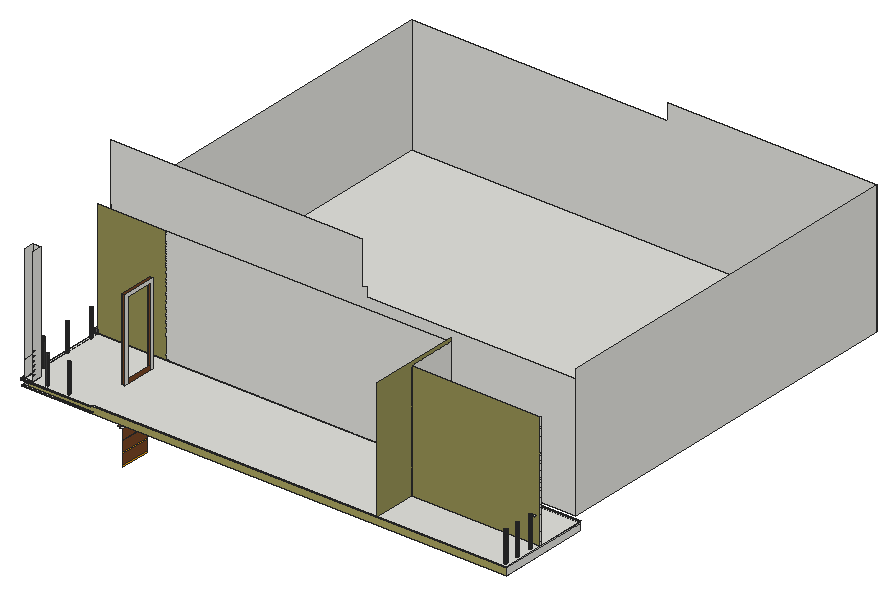
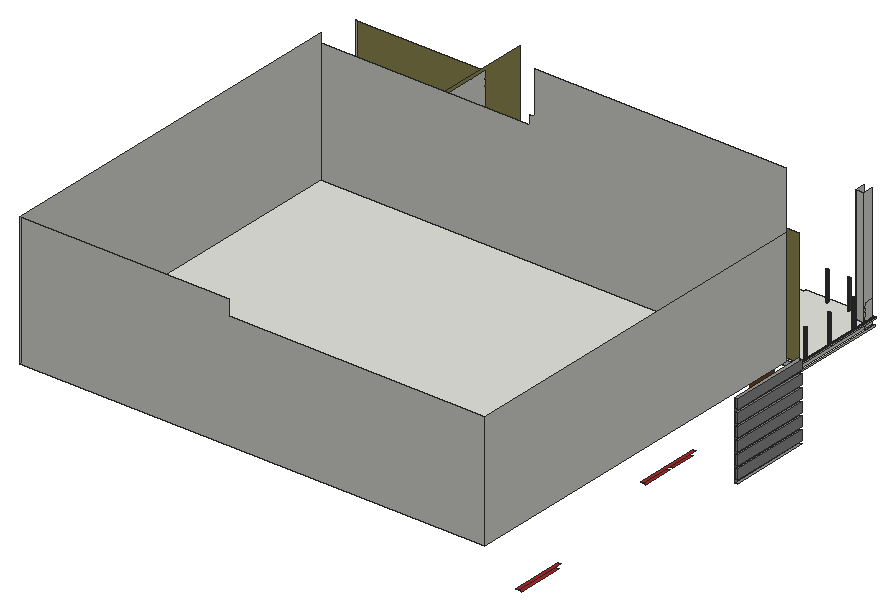
# SketchUp Ruby script. Lengths in inches.
U = 1.inch
M = Sketchup.active_model
def pt(a) = Geom::Point3d.new(a.map { |v| v * U })
def face(e, loops, mat)
  f = e.add_face(loops[0].map { |a| pt(a) })
  loops[1..].each { |l| e.add_face(l.map { |a| pt(a) }).erase! }
  f.material = f.back_material = mat if mat
  f
end
# faces: each face lists its corners as indices into pts; further lists are holes
def faces(e, pts, list, mat = nil) = list.each { |f| face(e, (f[0].is_a?(Array) ? f : [f]).map { |l| l.map { |i| pts[i] } }, mat) }
# xy, xz, yz: faces in a plane at the given z, y or x. An outline is a flat list of corners, or four numbers for a rectangle; further outlines are holes
def ring(l) = l.size == 4 ? [[l[0], l[1]], [l[2], l[1]], [l[2], l[3]], [l[0], l[3]]] : l.each_slice(2).to_a
def flat(e, list, mat, &to3) = list.each { |f| face(e, (f[0].is_a?(Array) ? f : [f]).map { |l| ring(l).map { |u, v| to3.(u, v) } }, mat) }
def xy(e, z, list, mat = nil) = flat(e, list, mat) { |x, y| [x, y, z] }
def xz(e, y, list, mat = nil) = flat(e, list, mat) { |x, z| [x, y, z] }
def yz(e, x, list, mat = nil) = flat(e, list, mat) { |y, z| [x, y, z] }
def lines(e, pts, list) = list.each { |a, b| e.add_line(pt(pts[a]), pt(pts[b])) }
# prism: a flat outline (further loops are holes) pulled along v
def prism(e, loops, v, mat = nil)
  f = face(e, loops, mat); d = Geom::Vector3d.new(v.map { |x| x * U })
  f.pushpull(f.normal.samedirection?(d) ? d.length : -d.length)
end
def box(e, o, s, mat = nil) = prism(e, [[o, [o[0] + s[0], o[1], o[2]], [o[0] + s[0], o[1] + s[1], o[2]], [o[0], o[1] + s[1], o[2]]]], [0, 0, s[2]], mat)
def at(x, y, z, deg = 0) = Geom::Transformation.translation(pt([x, y, z])) * Geom::Transformation.rotation(ORIGIN, Z_AXIS, deg.degrees)
def axes(o, x, y, z) = Geom::Transformation.new([*x, 0, *y, 0, *z, 0, *pt(o).to_a, 1])
def part(name) = M.definitions.add(name)
# library, detail: a bought-in or finely detailed component or shape, given as its bounding box
def library(name, o, s) = part(name).tap { |d| box(d.entities, o, s) }
def detail(e, o, s) = box(e.add_group.entities, o, s)
def put(e, d, t, mat = nil) = e.add_instance(d, t).tap { |i| i.material = mat if mat }
def group(e, t, mat = nil) = e.add_group.tap { |g| g.transformation = t; g.material = mat if mat }.entities
root = M.entities
M.materials.add("[0018_Brown]").color = [165, 42, 42]
M.materials.add("[0038_Orange]").color = [255, 165, 0]
M.materials.add("[0057_DarkKhaki]").color = [150, 145, 85]
M.materials.add("[0134_DimGray]").color = [105, 105, 105]
M.materials.add("[0137_Black]").color = [71, 71, 71]
M.materials.add("[Color M05]").color = [145, 145, 145]
M.materials.add("[Wood Veneer 01]").color = [120, 70, 37]
xy(root,168.28,[[8.875,116.75,11.875,199.5]],"[Color M05]")
xy(root,171.32,[[8.875,116.75,11.875,199.5]],"[Color M05]")
xy(root,181.4,[[8.875,116.75,11.875,199.5]],"[Color M05]")
xy(root,184.44,[[8.875,116.75,11.875,199.5]],"[Color M05]")
xy(root,191.21,[[8.875,431.78,11.875,479.72]],"[0018_Brown]")
xy(root,194.21,[[8.875,428.78,11.875,482.72]],"[0018_Brown]")
xy(root,194.53,[[8.875,116.75,11.875,199.5]],"[Color M05]")
xy(root,197.57,[[8.875,116.75,11.875,199.5]],"[Color M05]")
xy(root,204,[[79.85,61.11,82.85,91.11]])
xy(root,207,[[79.85,58.11,82.85,94.11]],"[Wood Veneer 01]")
xy(root,207.65,[[8.875,116.75,11.875,199.5]],"[Color M05]")
xy(root,210.69,[[8.875,116.75,11.875,199.5]],"[Color M05]")
xy(root,219.65,[[8.875,257.47,11.875,284.27],[8.875,287.91,11.875,318.35]],"[0018_Brown]")
xy(root,220.78,[[8.875,116.75,11.875,199.5]],"[Color M05]")
xy(root,222.65,[[8.875,254.47,11.875,321.35]],"[0018_Brown]")
xy(root,223.82,[[8.875,116.75,11.875,199.5]],"[Color M05]")
xy(root,233.9,[[8.875,116.75,11.875,199.5]],"[Color M05]")
xy(root,235.42,[[9.5625,21.375,9.5625,116.75,510.6875,116.75,510.6875,22.0625,82.9375,22.0625,82.9375,21.375]],"[0057_DarkKhaki]")
xy(root,236.47,[[9.5625,21.375,82.9375,21.375,82.9375,22.0625,11.875,22.0625,11.875,116.75,9.5625,116.75]])
xy(root,236.94,[[8.875,116.75,11.875,199.5]],"[Color M05]")
xy(root,242.04,[[20.875,22.0625,20.875,31.0625,11.875,31.0625,11.875,116.75,510.6875,116.75,510.6875,22.0625]])
xy(root,242.08,[[9.5625,19.6875,9.5625,116.75,11.875,116.75,11.875,22.0625,82.85,22.0625,82.85,19.6875]])
xy(root,243,[[9.5625,19.6875,9.5625,116.75,11.875,116.75,11.875,22.0625,82.85,22.0625,82.85,19.6875],[20.875,22.0625,82.85,22.0625,82.85,63.65,79.85,63.65,79.85,66.65,82.85,66.65,82.85,96.65,79.85,96.65,79.85,99.65,82.85,99.65,82.85,116.75,11.875,116.75,11.875,31.0625,20.875,31.0625],[376.99,22.0625,510.6875,66.25],[79.85,63.65,82.85,66.65],[376.99,66.25,509.75,116.75],
  [509.75,66.25,510.6875,116.75],[79.85,96.65,82.85,99.65],[11.875,116.75,376.99,119.6875],[376.99,116.75,509.75,119.6875],[20.875,122.75,501.6875,511.875]])
xy(root,243.17,[[[9.5625,19.6875,82.85,19.6875,82.85,22.0625,510.6875,22.0625,510.6875,116.75,9.5625,116.75],[11.875,22.0625,20.6875,32.5],[505.89,26.06,505.51,26.11,505.17,26.25,504.87,26.48,504.64,26.78,504.5,27.125,504.45,27.5,504.5,27.87,504.64,28.22,504.87,28.51,505.17,28.74,505.51,28.89,505.89,28.93,506.26,28.89,506.6,28.74,506.9,28.51,507.13,28.22,507.27,27.87,507.32,27.5,507.27,27.125,507.13,26.78,506.9,26.48,506.6,26.25,506.26,26.11],[505.89,40.75,505.51,40.8,505.17,40.9375,504.87,41.17,504.64,41.47,504.5,41.8125,504.45,42.18,504.5,42.56,504.64,42.9,504.87,43.2,505.17,43.43,505.51,43.57,505.89,43.62,506.26,43.57,506.6,43.43,506.9,43.2,507.13,42.9,507.27,42.56,507.32,42.18,507.27,41.8125,507.13,41.47,506.9,41.17,506.6,40.9375,506.26,40.8],[505.89,57.31,505.51,57.36,505.17,57.5,504.87,57.73,504.64,58.03,504.5,58.375,504.45,58.75,504.5,59.12,504.64,59.47,504.87,59.76,505.17,59.99,505.51,60.14,505.89,60.18,506.26,60.14,506.6,59.99,506.9,59.76,507.13,59.47,507.27,59.12,507.32,58.75,507.27,58.375,507.13,58.03,506.9,57.73,506.6,57.5,506.26,57.36],[12.37,75.91,12.03,75.99,11.73,76.14,11.48,76.375,11.29,76.67,11.19,76.99,11.18,77.34,11.25,77.67,11.41,77.97,11.65,78.23,11.9375,78.41,12.26,78.51,12.61,78.52,12.9375,78.45,13.24,78.29,13.49,78.06,13.68,77.77,13.78,77.44,13.79,77.1,13.72,76.76,13.56,76.46,13.33,76.21,13.04,76.03,12.71,75.92],[12.37,106.53,12.03,106.61,11.73,106.77,11.48,107,11.29,107.29,11.19,107.62,11.18,107.96,11.25,108.3,11.41,108.6,11.65,108.85,11.9375,109.03,12.26,109.14,12.61,109.15,12.9375,109.07,13.24,108.91,13.49,108.68,13.68,108.39,13.78,108.07,13.79,107.72,13.72,107.39,13.56,107.09,13.33,106.83,13.04,106.65,12.71,106.55],[12.37,43.72,12.03,43.8,11.73,43.96,11.48,44.1875,11.29,44.48,11.19,44.81,11.18,45.15,11.25,45.48,11.41,45.79,11.65,46.04,11.9375,46.22,12.26,46.32,12.61,46.34,12.9375,46.26,13.24,46.1,13.49,45.87,13.68,45.58,13.78,45.25,13.79,44.91,13.72,44.58,13.56,44.27,13.33,44.02,13.04,43.84,12.71,43.74],[56.47,23.05,56.16,23.09,55.875,23.21,55.63,23.39,55.44,23.64,55.32,23.93,55.28,24.23,55.32,24.54,55.44,24.83,55.63,25.07,55.875,25.26,56.16,25.38,56.47,25.42,56.78,25.38,57.0625,25.26,57.31,25.07,57.5,24.83,57.61,24.54,57.66,24.23,57.61,23.93,57.5,23.64,57.31,23.39,57.0625,23.21,56.78,23.09],[34.4,22.66,34.09,22.71,33.8,22.82,33.56,23.01,33.37,23.26,33.25,23.54,33.21,23.85,33.25,24.16,33.37,24.45,33.56,24.69,33.8,24.88,34.09,25,34.4,25.04,34.7,25,34.99,24.88,35.24,24.69,35.43,24.45,35.54,24.16,35.58,23.85,35.54,23.54,35.43,23.26,35.24,23.01,34.99,22.82,34.7,22.71]],[11.875,22.0625,20.6875,32.5]])
xz(root,31.0625,[[11.875,242.04,20.875,243]])
xz(root,32.5,[[11.875,243.17,20.6875,363.17]])
xz(root,63.65,[[79.85,243,82.85,327]],"[Wood Veneer 01]")
xz(root,66.25,[[509.75,243,510.6875,363]])
xz(root,66.25,[[[376.99,243,509.75,363],[504.58,267.58,504.11,267.64,503.67,267.83,503.3,268.11,503.01,268.49,502.83,268.93,502.77,269.39,502.83,269.86,503.01,270.3,503.3,270.68,503.67,270.96,504.11,271.15,504.58,271.21,505.05,271.15,505.49,270.96,505.86,270.68,506.15,270.3,506.33,269.86,506.39,269.39,506.33,268.93,506.15,268.49,505.86,268.11,505.49,267.83,505.05,267.64]]],"[0057_DarkKhaki]")
xz(root,66.65,[[79.85,243,82.85,324]],"[Wood Veneer 01]")
xz(root,96.65,[[79.85,243,82.85,324]],"[Wood Veneer 01]")
xz(root,99.65,[[79.85,243,82.85,327]],"[Wood Veneer 01]")
xz(root,116.75,[[9.5625,235.42,11.875,236.47],[11.875,235.42,82.85,242.04],[82.85,235.42,376.99,242.04],[376.99,235.42,509.75,242.04],[509.75,235.42,510.6875,242.04],
  [8.875,236.94,11.875,242.04],[8.875,242.04,11.875,242.08],[11.875,242.04,82.85,243],[82.85,242.04,376.99,243],[376.99,242.04,509.75,243],
  [509.75,242.04,510.6875,243],[8.875,242.08,9.5625,243],[9.5625,242.08,11.875,243],[8.875,243,9.5625,243.17],[9.5625,243,11.875,243.17],
  [11.875,243,82.85,243.17],[82.85,243,376.99,243.17],[376.99,243,509.75,243.17],[509.75,243,510.6875,243.17],[82.85,243.17,376.99,363]])
xz(root,116.75,[[11.875,243.17,82.85,363.37]],"[0057_DarkKhaki]")
xz(root,116.75,[[8.875,171.32,11.875,181.4],[8.875,184.44,11.875,194.53],[8.875,197.57,11.875,207.65],[8.875,210.69,11.875,220.78],[8.875,223.82,11.875,233.9],
  [8.875,243.17,11.875,247.03]],"[0134_DimGray]")
xz(root,122.75,[[20.875,243,20.875,423,281.04,423,281.04,379.43,285.29,379.43,285.29,369.99,501.6875,369.99,501.6875,243]])
xz(root,199.5,[[8.875,171.32,11.875,181.4],[8.875,184.44,11.875,194.53],[8.875,197.57,11.875,207.65],[8.875,210.69,11.875,220.78],[8.875,223.82,11.875,233.9],
  [8.875,236.94,11.875,247.03]],"[Color M05]")
xz(root,511.875,[[20.875,243,501.6875,243,501.6875,379.43,286.17,379.43,286.17,363,20.875,363]])
yz(root,8.875,[[116.75,171.32,199.5,181.4],[116.75,184.44,199.5,194.53],[116.75,197.57,199.5,207.65],[116.75,210.69,199.5,220.78],[116.75,223.82,199.5,233.9],
  [116.75,236.94,199.5,247.03]],"[Color M05]")
yz(root,9.5625,[[21.375,235.42,116.75,236.47],[19.6875,242.08,116.75,243],[19.6875,243,116.75,243.17]])
yz(root,11.875,[[116.75,171.32,199.5,181.4],[116.75,184.44,199.5,194.53],[116.75,197.57,199.5,207.65],[116.75,210.69,199.5,220.78],[116.75,223.82,199.5,233.9],
  [22.0625,235.42,31.0625,236.47],[22.0625,236.47,31.0625,242.04],[31.0625,236.47,116.75,242.04],[116.75,236.94,199.5,247.03],[22.0625,242.04,31.0625,242.08],
  [31.0625,242.04,116.75,242.08],[22.0625,242.08,31.0625,243],[31.0625,242.08,116.75,243],[22.0625,243,31.0625,243.17],[22.0625,243.17,31.0625,260.5],
  [31.0625,243.17,31.0625,260.5,22.0625,260.5,22.0625,363.17,32.5,363.17,32.5,243.17]])
yz(root,11.875,[[116.75,168.28,199.5,171.32],[116.75,181.4,199.5,184.44],[116.75,194.53,199.5,197.57],[116.75,207.65,199.5,210.69],[116.75,220.78,199.5,223.82],
  [116.75,233.9,199.5,236.94]],"[Color M05]")
yz(root,20.6875,[[22.0625,243.17,32.5,243.17,32.5,363.17,22.0625,363.17,22.0625,270.71,22.23,271.12,22.5,271.47,22.85,271.74,23.26,271.91,23.69,271.96,24.13,271.91,24.54,271.74,24.89,271.47,25.15,271.12,25.32,270.71,25.38,270.28,25.32,269.84,25.15,269.43,24.89,269.08,24.54,268.8125,24.13,268.65,23.69,268.59,23.26,268.65,22.85,268.8125,22.5,269.08,22.23,269.43,22.0625,269.84,22.0625,266.27,22.23,266.68,22.5,267.03,22.85,267.3,23.26,267.47,23.69,267.53,24.13,267.47,24.54,267.3,24.89,267.03,25.15,266.68,25.32,266.27,25.38,265.84,25.32,265.4,25.15,264.99,24.89,264.64,24.54,264.375,24.13,264.21,23.69,264.15,23.26,264.21,22.85,264.375,22.5,264.64,22.23,264.99,22.0625,265.4,22.0625,261.84,22.23,262.24,22.5,262.59,22.85,262.86,23.26,263.03,23.69,263.09,24.13,263.03,24.54,262.86,24.89,262.59,25.15,262.24,25.32,261.84,25.38,261.4,25.32,260.96,25.15,260.56,24.89,260.21,24.54,259.9375,24.13,259.77,23.69,259.71,23.26,259.77,22.85,259.9375,22.5,260.21,22.23,260.56,22.0625,260.96,22.0625,257.4,22.23,257.81,22.5,258.16,22.85,258.42,23.26,258.59,23.69,258.65,24.13,258.59,24.54,258.42,24.89,258.16,25.15,257.81,25.32,257.4,25.38,256.96,25.32,256.53,25.15,256.12,24.89,255.77,24.54,255.5,24.13,255.33,23.69,255.28,23.26,255.33,22.85,255.5,22.5,255.77,22.23,256.12,22.0625,256.53,22.0625,252.96,22.23,253.37,22.5,253.72,22.85,253.99,23.26,254.16,23.69,254.21,24.13,254.16,24.54,253.99,24.89,253.72,25.15,253.37,25.32,252.96,25.38,252.53,25.32,252.09,25.15,251.68,24.89,251.33,24.54,251.0625,24.13,250.9,23.69,250.84,23.26,250.9,22.85,251.0625,22.5,251.33,22.23,251.68,22.0625,252.09,22.0625,248.52,22.23,248.93,22.5,249.28,22.85,249.55,23.26,249.72,23.69,249.78,24.13,249.72,24.54,249.55,24.89,249.28,25.15,248.93,25.32,248.52,25.38,248.09,25.32,247.65,25.15,247.24,24.89,246.89,24.54,246.625,24.13,246.46,23.69,246.4,23.26,246.46,22.85,246.625,22.5,246.89,22.23,247.24,22.0625,247.65]])
yz(root,20.875,[[22.0625,242.04,31.0625,243],[122.75,243,511.875,363]])
yz(root,79.85,[[63.65,243,63.65,327,99.65,327,99.65,243,96.65,243,96.65,324,66.65,324,66.65,243]],"[Wood Veneer 01]")
yz(root,82.85,[[63.65,243,66.65,243,66.65,324,96.65,324,96.65,243,99.65,243,99.65,327,63.65,327]])
yz(root,82.85,[[61.11,168.92,91.11,170.17],[61.11,180.86,91.11,182.11],[61.11,192.8,91.11,194.05]],"[0038_Orange]")
yz(root,82.85,[[61.11,170.17,91.11,180.86],[61.11,182.11,91.11,192.8],[61.11,194.05,91.11,204],[66.65,243,96.65,247.86]],"[Wood Veneer 01]")
yz(root,376.99,[[66.25,243,116.75,363]])
yz(root,376.99,[[22.0625,243,66.25,243,66.25,363,116.75,363,116.75,367,22.0625,367]],"[0057_DarkKhaki]")
yz(root,501.6875,[[122.75,243,511.875,379.43]])
yz(root,510.6875,[[22.0625,235.42,116.75,242.04],[22.0625,242.04,66.25,243],[66.25,242.04,116.75,243],[22.0625,243,66.25,243.17],[66.25,243,116.75,243.17]])
p = [[35.43,23.26,243.17],[35.54,23.54,243.17],[35.54,23.54,272.92],[35.43,23.26,272.92],[55.44,23.64,243.17],[55.63,23.39,243.17],
  [55.63,23.39,272.92],[55.44,23.64,272.92],[57.31,23.39,243.17],[57.5,23.64,243.17],[57.5,23.64,272.92],[57.31,23.39,272.92],
  [33.21,23.85,243.17],[33.25,23.54,243.17],[33.25,23.54,272.92],[33.21,23.85,272.92],[35.58,23.85,243.17],[35.58,23.85,272.92],
  [55.32,23.93,243.17],[55.32,23.93,272.92],[57.61,23.93,243.17],[57.61,23.93,272.92],[33.25,24.16,243.17],[33.25,24.16,272.92],
  [35.54,24.16,243.17],[35.54,24.16,272.92],[55.28,24.23,243.17],[55.28,24.23,272.92],[57.66,24.23,243.17],[57.66,24.23,272.92],
  [33.37,24.45,243.17],[33.37,24.45,272.92],[35.43,24.45,243.17],[35.43,24.45,272.92],[55.32,24.54,243.17],[55.32,24.54,272.92],
  [57.61,24.54,243.17],[57.61,24.54,272.92],[33.56,24.69,243.17],[33.56,24.69,272.92],[35.24,24.69,243.17],[35.24,24.69,272.92],
  [55.44,24.83,243.17],[55.44,24.83,272.92],[57.5,24.83,243.17],[57.5,24.83,272.92],[33.8,24.88,243.17],[33.8,24.88,272.92],
  [34.99,24.88,243.17],[34.99,24.88,272.92],[55.63,25.07,243.17],[55.63,25.07,272.92],[57.31,25.07,243.17],[57.31,25.07,272.92],
  [34.09,25,243.17],[34.09,25,272.92],[34.7,25,243.17],[34.7,25,272.92],[34.4,25.04,243.17],[34.4,25.04,272.92],
  [55.875,25.26,243.17],[55.875,25.26,272.92],[57.0625,25.26,243.17],[57.0625,25.26,272.92],[56.16,25.38,243.17],[56.16,25.38,272.92],
  [56.78,25.38,243.17],[56.78,25.38,272.92],[56.47,25.42,243.17],[56.47,25.42,272.92],[505.17,26.25,243.17],[505.51,26.11,243.17],
  [505.51,26.11,274.04],[505.17,26.25,274.04],[505.89,26.06,243.17],[505.89,26.06,274.04],[506.26,26.11,243.17],[506.26,26.11,274.04],
  [506.6,26.25,243.17],[506.6,26.25,274.04],[504.87,26.48,243.17],[504.87,26.48,274.04],[506.9,26.48,243.17],[506.9,26.48,274.04],
  [504.64,26.78,243.17],[504.64,26.78,274.04],[507.13,26.78,243.17],[507.13,26.78,274.04],[504.5,27.125,243.17],[504.5,27.125,274.04],
  [507.27,27.125,243.17],[507.27,27.125,274.04],[504.45,27.5,243.17],[504.45,27.5,274.04],[507.32,27.5,243.17],[507.32,27.5,274.04],
  [504.5,27.87,243.17],[504.5,27.87,274.04],[507.27,27.87,243.17],[507.27,27.87,274.04],[504.64,28.22,243.17],[504.64,28.22,274.04],
  [507.13,28.22,243.17],[507.13,28.22,274.04],[504.87,28.51,243.17],[504.87,28.51,274.04],[506.9,28.51,243.17],[506.9,28.51,274.04],
  [505.17,28.74,243.17],[505.17,28.74,274.04],[506.6,28.74,243.17],[506.6,28.74,274.04],[505.51,28.89,243.17],[505.51,28.89,274.04],
  [506.26,28.89,243.17],[506.26,28.89,274.04],[505.89,28.93,243.17],[505.89,28.93,274.04],[505.51,40.8,243.17],[505.89,40.75,243.17],
  [505.89,40.75,274.04],[505.51,40.8,274.04],[506.26,40.8,243.17],[506.26,40.8,274.04],[505.17,40.9375,243.17],[505.17,40.9375,274.04],
  [506.6,40.9375,243.17],[506.6,40.9375,274.04],[504.87,41.17,243.17],[504.87,41.17,274.04],[506.9,41.17,243.17],[506.9,41.17,274.04],
  [504.64,41.47,243.17],[504.64,41.47,274.04],[507.13,41.47,243.17],[507.13,41.47,274.04],[504.5,41.8125,243.17],[504.5,41.8125,274.04],
  [507.27,41.8125,243.17],[507.27,41.8125,274.04],[504.45,42.18,243.17],[504.45,42.18,274.04],[507.32,42.18,243.17],[507.32,42.18,274.04],
  [504.5,42.56,243.17],[504.5,42.56,274.04],[507.27,42.56,243.17],[507.27,42.56,274.04],[504.64,42.9,243.17],[504.64,42.9,274.04],
  [507.13,42.9,243.17],[507.13,42.9,274.04],[504.87,43.2,243.17],[504.87,43.2,274.04],[506.9,43.2,243.17],[506.9,43.2,274.04],
  [505.17,43.43,243.17],[505.17,43.43,274.04],[506.6,43.43,243.17],[506.6,43.43,274.04],[505.51,43.57,243.17],[505.51,43.57,274.04],
  [506.26,43.57,243.17],[506.26,43.57,274.04],[505.89,43.62,243.17],[505.89,43.62,274.04],[12.03,43.8,243.17],[12.37,43.72,243.17],
  [12.37,43.72,271.42],[12.03,43.8,271.42],[12.71,43.74,243.17],[12.71,43.74,271.42],[13.04,43.84,243.17],[13.04,43.84,271.42],
  [11.73,43.96,243.17],[11.73,43.96,271.42],[13.33,44.02,243.17],[13.33,44.02,271.42],[11.48,44.1875,243.17],[11.48,44.1875,271.42],
  [13.56,44.27,243.17],[13.56,44.27,271.42],[11.29,44.48,243.17],[11.29,44.48,271.42],[13.72,44.58,243.17],[13.72,44.58,271.42],
  [11.19,44.81,243.17],[11.19,44.81,271.42],[13.79,44.91,243.17],[13.79,44.91,271.42],[11.18,45.15,243.17],[11.18,45.15,271.42],
  [13.78,45.25,243.17],[13.78,45.25,271.42],[11.25,45.48,243.17],[11.25,45.48,271.42],[13.68,45.58,243.17],[13.68,45.58,271.42],
  [11.41,45.79,243.17],[11.41,45.79,271.42],[13.49,45.87,243.17],[13.49,45.87,271.42],[11.65,46.04,243.17],[11.65,46.04,271.42],
  [13.24,46.1,243.17],[13.24,46.1,271.42],[11.9375,46.22,243.17],[11.9375,46.22,271.42],[12.9375,46.26,243.17],[12.9375,46.26,271.42],
  [12.26,46.32,243.17],[12.26,46.32,271.42],[12.61,46.34,243.17],[12.61,46.34,271.42],[505.51,57.36,243.17],[505.89,57.31,243.17],
  [505.89,57.31,274.04],[505.51,57.36,274.04],[506.26,57.36,243.17],[506.26,57.36,274.04],[505.17,57.5,243.17],[505.17,57.5,274.04],
  [506.6,57.5,243.17],[506.6,57.5,274.04],[504.87,57.73,243.17],[504.87,57.73,274.04],[506.9,57.73,243.17],[506.9,57.73,274.04],
  [504.64,58.03,243.17],[504.64,58.03,274.04],[507.13,58.03,243.17],[507.13,58.03,274.04],[504.5,58.375,243.17],[504.5,58.375,274.04],
  [507.27,58.375,243.17],[507.27,58.375,274.04],[504.45,58.75,243.17],[504.45,58.75,274.04],[507.32,58.75,243.17],[507.32,58.75,274.04],
  [504.5,59.12,243.17],[504.5,59.12,274.04],[507.27,59.12,243.17],[507.27,59.12,274.04],[504.64,59.47,243.17],[504.64,59.47,274.04],
  [507.13,59.47,243.17],[507.13,59.47,274.04],[504.87,59.76,243.17],[504.87,59.76,274.04],[506.9,59.76,243.17],[506.9,59.76,274.04],
  [505.17,59.99,243.17],[505.17,59.99,274.04],[506.6,59.99,243.17],[506.6,59.99,274.04],[505.51,60.14,243.17],[505.51,60.14,274.04],
  [506.26,60.14,243.17],[506.26,60.14,274.04],[505.89,60.18,243.17],[505.89,60.18,274.04],[12.03,75.99,243.17],[12.37,75.91,243.17],
  [12.37,75.91,271.42],[12.03,75.99,271.42],[12.71,75.92,243.17],[12.71,75.92,271.42],[13.04,76.03,243.17],[13.04,76.03,271.42],
  [11.73,76.14,243.17],[11.73,76.14,271.42],[13.33,76.21,243.17],[13.33,76.21,271.42],[11.48,76.375,243.17],[11.48,76.375,271.42],
  [13.56,76.46,243.17],[13.56,76.46,271.42],[11.29,76.67,243.17],[11.29,76.67,271.42],[13.72,76.76,243.17],[13.72,76.76,271.42],
  [11.19,76.99,243.17],[11.19,76.99,271.42],[13.79,77.1,243.17],[13.79,77.1,271.42],[11.18,77.34,243.17],[11.18,77.34,271.42],
  [13.78,77.44,243.17],[13.78,77.44,271.42],[11.25,77.67,243.17],[11.25,77.67,271.42],[13.68,77.77,243.17],[13.68,77.77,271.42],
  [11.41,77.97,243.17],[11.41,77.97,271.42],[13.49,78.06,243.17],[13.49,78.06,271.42],[11.65,78.23,243.17],[11.65,78.23,271.42],
  [13.24,78.29,243.17],[13.24,78.29,271.42],[11.9375,78.41,243.17],[11.9375,78.41,271.42],[12.9375,78.45,243.17],[12.9375,78.45,271.42],
  [12.26,78.51,243.17],[12.26,78.51,271.42],[12.61,78.52,243.17],[12.61,78.52,271.42],[12.03,106.61,243.17],[12.37,106.53,243.17],
  [12.37,106.53,271.42],[12.03,106.61,271.42],[12.71,106.55,243.17],[12.71,106.55,271.42],[13.04,106.65,243.17],[13.04,106.65,271.42],
  [11.73,106.77,243.17],[11.73,106.77,271.42],[13.33,106.83,243.17],[13.33,106.83,271.42],[11.48,107,243.17],[11.48,107,271.42],
  [13.56,107.09,243.17],[13.56,107.09,271.42],[11.29,107.29,243.17],[11.29,107.29,271.42],[13.72,107.39,243.17],[13.72,107.39,271.42],
  [11.19,107.62,243.17],[11.19,107.62,271.42],[13.79,107.72,243.17],[13.79,107.72,271.42],[11.18,107.96,243.17],[11.18,107.96,271.42],
  [13.78,108.07,243.17],[13.78,108.07,271.42],[11.25,108.3,243.17],[11.25,108.3,271.42],[13.68,108.39,243.17],[13.68,108.39,271.42],
  [11.41,108.6,243.17],[11.41,108.6,271.42],[13.49,108.68,243.17],[13.49,108.68,271.42],[11.65,108.85,243.17],[11.65,108.85,271.42],
  [13.24,108.91,243.17],[13.24,108.91,271.42],[11.9375,109.03,243.17],[11.9375,109.03,271.42],[12.9375,109.07,243.17],[12.9375,109.07,271.42],
  [12.26,109.14,243.17],[12.26,109.14,271.42],[12.61,109.15,243.17],[12.61,109.15,271.42]]
faces(root,p,[[0,1,2,3],[4,5,6,7],[8,9,10,11],[12,13,14,15],[1,16,17,2],[18,4,7,19],[9,20,21,10],[22,12,15,23],
  [16,24,25,17],[26,18,19,27],[20,28,29,21],[30,22,23,31],[24,32,33,25],[34,26,27,35],[28,36,37,29],[38,30,31,39],
  [32,40,41,33],[42,34,35,43],[36,44,45,37],[46,38,39,47],[40,48,49,41],[50,42,43,51],[44,52,53,45],[54,46,47,55],
  [48,56,57,49],[58,54,55,59],[56,58,59,57],[60,50,51,61],[52,62,63,53],[64,60,61,65],[62,66,67,63],[68,64,65,69],
  [66,68,69,67],[70,71,72,73],[71,74,75,72],[74,76,77,75],[76,78,79,77],[80,70,73,81],[78,82,83,79],[84,80,81,85],
  [82,86,87,83],[88,84,85,89],[86,90,91,87],[92,88,89,93],[90,94,95,91],[96,92,93,97],[94,98,99,95],[100,96,97,101],
  [98,102,103,99],[104,100,101,105],[102,106,107,103],[108,104,105,109],[106,110,111,107],[112,108,109,113],[110,114,115,111],[116,112,113,117],
  [114,116,117,115],[118,119,120,121],[119,122,123,120],[124,118,121,125],[122,126,127,123],[128,124,125,129],[126,130,131,127],[132,128,129,133],
  [130,134,135,131],[136,132,133,137],[134,138,139,135],[140,136,137,141],[138,142,143,139],[144,140,141,145],[142,146,147,143],[148,144,145,149],
  [146,150,151,147],[152,148,149,153],[150,154,155,151],[156,152,153,157],[154,158,159,155],[160,156,157,161],[158,162,163,159],[164,160,161,165],
  [162,164,165,163],[166,167,168,169],[167,170,171,168],[170,172,173,171],[174,166,169,175],[172,176,177,173],[178,174,175,179],[176,180,181,177],
  [182,178,179,183],[180,184,185,181],[186,182,183,187],[184,188,189,185],[190,186,187,191],[188,192,193,189],[194,190,191,195],[192,196,197,193],
  [198,194,195,199],[196,200,201,197],[202,198,199,203],[200,204,205,201],[206,202,203,207],[204,208,209,205],[210,206,207,211],[212,210,211,213],
  [208,212,213,209],[214,215,216,217],[215,218,219,216],[220,214,217,221],[218,222,223,219],[224,220,221,225],[222,226,227,223],[228,224,225,229],
  [226,230,231,227],[232,228,229,233],[230,234,235,231],[236,232,233,237],[234,238,239,235],[240,236,237,241],[238,242,243,239],[244,240,241,245],
  [242,246,247,243],[248,244,245,249],[246,250,251,247],[252,248,249,253],[250,254,255,251],[256,252,253,257],[254,258,259,255],[260,256,257,261],
  [258,260,261,259],[262,263,264,265],[263,266,267,264],[266,268,269,267],[270,262,265,271],[268,272,273,269],[274,270,271,275],[272,276,277,273],
  [278,274,275,279],[276,280,281,277],[282,278,279,283],[280,284,285,281],[286,282,283,287],[284,288,289,285],[290,286,287,291],[288,292,293,289],
  [294,290,291,295],[292,296,297,293],[298,294,295,299],[296,300,301,297],[302,298,299,303],[300,304,305,301],[306,302,303,307],[304,308,309,305],
  [308,306,307,309],[310,311,312,313],[311,314,315,312],[314,316,317,315],[318,310,313,319],[316,320,321,317],[322,318,319,323],[320,324,325,321],
  [326,322,323,327],[324,328,329,325],[330,326,327,331],[328,332,333,329],[334,330,331,335],[332,336,337,333],[338,334,335,339],[336,340,341,337],
  [342,338,339,343],[340,344,345,341],[346,342,343,347],[344,348,349,345],[350,346,347,351],[348,352,353,349],[354,350,351,355],[356,354,355,357],
  [352,356,357,353]],"[0137_Black]")
